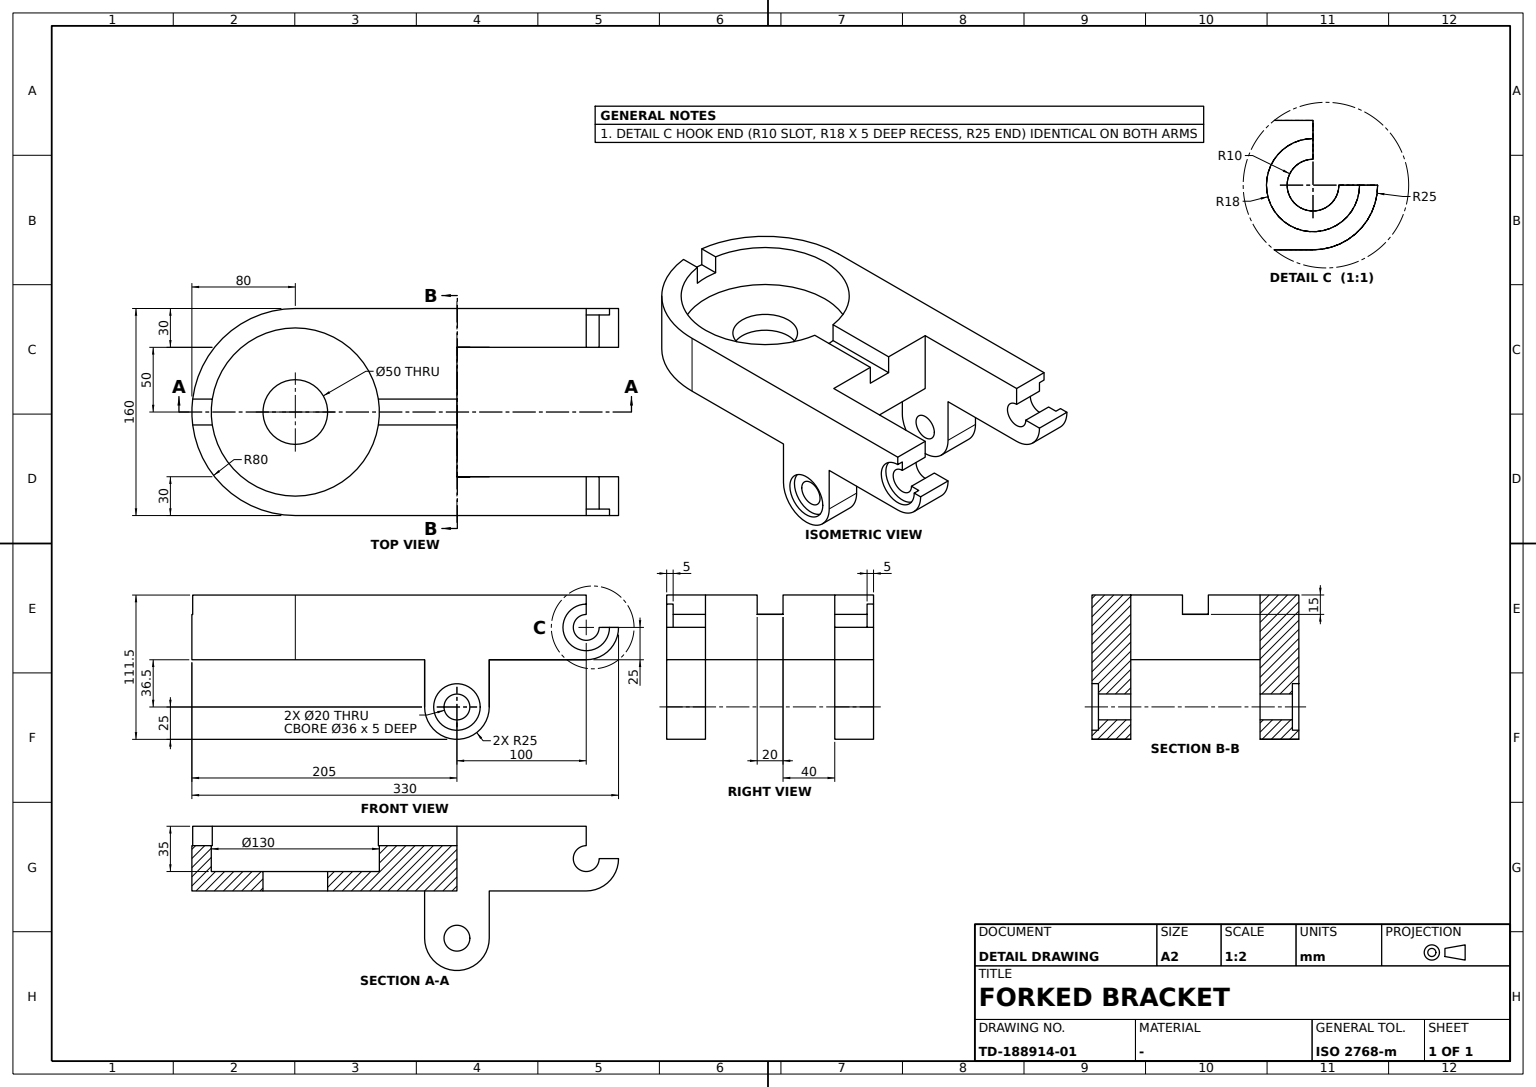
solid
v1 (75,107,25)
v2 (75,143,25)
e1 v1 v2 CIRCLE(AX(P(75,125,25),D(1,0,0),D(0,1,0)),18)
v3 (80,107,25)
e2 v3 v1 LINE
v4 (80,143,25)
e3 v3 v4 CIRCLE(AX(P(80,125,25),D(1,0,0),D(0,1,0)),18)
e4 v4 v2 LINE
face CYL(AX(P(77.5,125,25),D(-1,0,0),D(0,1,0)),18) rev [-e1 -e2 e3 e4]
v5 (-80,0,-36.5)
v6 (-80,50,-36.5)
e5 v5 v6 CIRCLE(AX(P(-80,25,-36.5),D(1,0,0),D(0,1,0)),25)
v7 (-50,50,-36.5)
e6 v6 v7 LINE
v8 (-50,0,-36.5)
e7 v7 v8 CIRCLE(AX(P(-50,25,-36.5),D(-1,0,0),D(0,1,0)),25)
e8 v5 v8 LINE
face CYL(AX(P(0,25,-36.5),D(-1,0,0),D(0,1,0)),25) [e5 e6 e7 -e8]
v9 (-80,125,43)
v10 (-80,125,50)
e9 v9 v10 LINE
v11 (-50,125,50)
e10 v11 v10 LINE
v12 (-50,125,35)
e11 v12 v11 LINE
v13 (-75,125,35)
e12 v12 v13 LINE
v14 (-75,125,43)
e13 v13 v14 LINE
e14 v14 v9 LINE
face PLANE(AX(P(80,125,25),D(0,-1,0),D(0,0,1))) rev [e9 -e10 -e11 e12 e13 e14]
v15 (-25,-100.000066,15)
v16 (-25,-100.000066,0)
e15 v15 v16 LINE
v17 (25,-100.000066,15)
e16 v15 v17 CIRCLE(AX(P(0,-100.000066,15),D(0,0,1),D(1,0,0)),25)
v18 (25,-100.000066,0)
e17 v17 v18 LINE
e18 v18 v16 CIRCLE(AX(P(0,-100.000066,0),D(0,0,-1),D(0,1,0)),25)
face CYL(AX(P(0,-100.000066,-2.5),D(0,0,-1),D(1,0,0)),25) rev [-e15 e16 e17 e18]
v19 (-50,50,0)
v20 (-50,125,0)
e19 v19 v20 LINE
v21 (-80,50,0)
e20 v21 v19 LINE
v22 (-80,125,0)
e21 v21 v22 LINE
e22 v20 v22 LINE
face PLANE(AX(P(0,50,0),D(0,0,-1),D(0,1,0))) [-e19 -e20 e21 -e22]
v23 (-80,107,25)
v24 (-80,143,25)
e23 v23 v24 CIRCLE(AX(P(-80,125,25),D(1,0,0),D(0,1,0)),18)
v25 (-75,107,25)
e24 v23 v25 LINE
v26 (-75,143,25)
e25 v25 v26 CIRCLE(AX(P(-75,125,25),D(1,0,0),D(0,1,0)),18)
e26 v24 v26 LINE
face CYL(AX(P(77.5,125,25),D(-1,0,0),D(0,1,0)),18) rev [-e23 e24 e25 -e26]
v27 (-80,150,25)
e27 v24 v27 LINE
v28 (-75,135,25)
e28 v28 v26 LINE
v29 (-50,135,25)
e29 v29 v28 LINE
v30 (-50,150,25)
e30 v29 v30 LINE
e31 v27 v30 LINE
face PLANE(AX(P(80,125,25),D(0,0,1),D(0,1,0))) [-e27 e26 -e28 -e29 e30 -e31]
v31 (75,15,-36.5)
v32 (50,15,-36.5)
e32 v31 v32 LINE
v33 (50,35,-36.5)
e33 v33 v32 CIRCLE(AX(P(50,25,-36.5),D(1,0,0),D(0,-1,0)),10)
v34 (75,35,-36.5)
e34 v34 v33 LINE
e35 v34 v31 CIRCLE(AX(P(75,25,-36.5),D(1,0,0),D(0,1,0)),10)
face CYL(AX(P(-0.66,25,-36.5),D(-1,0,0),D(0,1,0)),10) rev [e32 -e33 -e34 e35]
e36 v14 v25 CIRCLE(AX(P(-75,125,25),D(1,0,0),D(0,1,0)),18)
e37 v9 v23 CIRCLE(AX(P(-80,125,25),D(1,0,0),D(0,1,0)),18)
face CYL(AX(P(77.5,125,25),D(-1,0,0),D(0,1,0)),18) rev [e36 -e24 -e37 -e14]
v35 (-75,115,25)
e38 v35 v28 CIRCLE(AX(P(-75,125,25),D(1,0,0),D(0,1,0)),10)
v36 (-50,115,25)
e39 v36 v35 LINE
e40 v29 v36 CIRCLE(AX(P(-50,125,25),D(-1,0,0),D(0,1,0)),10)
face CYL(AX(P(-3.16,125,25),D(-1,0,0),D(0,1,0)),10) rev [-e38 -e39 -e40 e29]
v37 (75,115,25)
v38 (50,115,25)
e41 v37 v38 LINE
v39 (75,135,25)
e42 v37 v39 CIRCLE(AX(P(75,125,25),D(1,0,0),D(0,1,0)),10)
v40 (50,135,25)
e43 v39 v40 LINE
e44 v38 v40 CIRCLE(AX(P(50,125,25),D(1,0,0),D(0,-1,0)),10)
face CYL(AX(P(-3.16,125,25),D(-1,0,0),D(0,1,0)),10) rev [-e41 e42 e43 -e44]
e45 v13 v35 CIRCLE(AX(P(-75,125,25),D(1,0,0),D(0,1,0)),10)
face PLANE(AX(P(-75,0,0),D(1,0,0),D(0,1,0))) rev [-e36 -e13 e45 e38 e28 -e25]
e46 v16 v18 CIRCLE(AX(P(0,-100.000066,0),D(0,0,-1),D(0,1,0)),25)
v41 (50,25,0)
v42 (50,0,0)
e47 v41 v42 LINE
v43 (80,0,0)
e48 v42 v43 LINE
v44 (80,-100,0)
e49 v44 v43 LINE
v45 (80,-100.000066,0)
e50 v45 v44 CIRCLE(AX(P(0,-100.000066,0),D(0,0,1),D(1,0,0)),80)
v46 (-80,-100.000066,0)
e51 v46 v45 CIRCLE(AX(P(0,-100.000066,0),D(0,0,1),D(1,0,0)),80)
v47 (-80,-100,0)
e52 v47 v46 CIRCLE(AX(P(0,-100.000066,0),D(0,0,1),D(1,0,0)),80)
v48 (-80,0,0)
e53 v47 v48 LINE
v49 (-50,0,0)
e54 v48 v49 LINE
v50 (-50,25,0)
e55 v50 v49 LINE
e56 v50 v41 LINE
face PLANE(AX(P(0,50,0),D(0,0,-1),D(0,1,0))) [-e18 -e46] [e47 e48 -e49 -e50 -e51 -e52 e53 e54 -e55 e56]
e57 v7 v19 LINE
e58 v6 v21 LINE
face PLANE(AX(P(0,50,-36.5),D(0,1,0),D(0,0,1))) [-e57 -e6 e58 e20]
e59 v32 v33 CIRCLE(AX(P(50,25,-36.5),D(1,0,0),D(0,-1,0)),10)
v51 (50,125,0)
v52 (50,150,25)
e60 v51 v52 CIRCLE(AX(P(50,125,25),D(1,0,0),D(0,1,0)),25)
v53 (50,50,0)
e61 v53 v51 LINE
v54 (50,50,-36.5)
e62 v54 v53 LINE
v55 (50,0,-36.5)
e63 v55 v54 CIRCLE(AX(P(50,25,-36.5),D(1,0,0),D(0,-1,0)),25)
e64 v42 v55 LINE
v56 (50,25,50)
e65 v56 v41 LINE
v57 (50,125,50)
e66 v56 v57 LINE
v58 (50,125,35)
e67 v58 v57 LINE
e68 v58 v38 CIRCLE(AX(P(50,125,25),D(1,0,0),D(0,-1,0)),10)
e69 v40 v52 LINE
face PLANE(AX(P(50,128.473083,50),D(1,0,0),D(0,-1,0))) rev [e59 e33] [-e60 -e61 -e62 -e63 -e64 -e47 -e65 e66 -e67 e68 e44 e69]
v59 (-75,43,-36.5)
v60 (-75,7,-36.5)
e70 v59 v60 CIRCLE(AX(P(-75,25,-36.5),D(1,0,0),D(0,1,0)),18)
v61 (-80,7,-36.5)
e71 v61 v60 LINE
v62 (-80,43,-36.5)
e72 v62 v61 CIRCLE(AX(P(-80,25,-36.5),D(1,0,0),D(0,1,0)),18)
e73 v62 v59 LINE
face CYL(AX(P(77.5,25,-36.5),D(-1,0,0),D(0,1,0)),18) rev [e70 -e71 -e72 e73]
v63 (80,50,-36.5)
e74 v54 v63 LINE
v64 (80,0,-36.5)
e75 v64 v63 CIRCLE(AX(P(80,25,-36.5),D(1,0,0),D(0,1,0)),25)
e76 v55 v64 LINE
face CYL(AX(P(0,25,-36.5),D(-1,0,0),D(0,1,0)),25) [e63 e74 -e75 -e76]
v65 (-50,15,-36.5)
v66 (-50,35,-36.5)
e77 v65 v66 CIRCLE(AX(P(-50,25,-36.5),D(-1,0,0),D(0,1,0)),10)
e78 v66 v65 CIRCLE(AX(P(-50,25,-36.5),D(-1,0,0),D(0,1,0)),10)
e79 v49 v8 LINE
e80 v20 v30 CIRCLE(AX(P(-50,125,25),D(1,0,0),D(0,1,0)),25)
e81 v36 v12 CIRCLE(AX(P(-50,125,25),D(-1,0,0),D(0,1,0)),10)
v67 (-50,25,50)
e82 v11 v67 LINE
e83 v67 v50 LINE
face PLANE(AX(P(-50,25,50),D(-1,0,0),D(0,1,0))) rev [e77 e78] [e55 e79 -e7 e57 e19 e80 -e30 e40 e81 e11 e82 e83]
v68 (-75,15,-36.5)
v69 (-75,35,-36.5)
e84 v68 v69 CIRCLE(AX(P(-75,25,-36.5),D(1,0,0),D(0,1,0)),10)
e85 v65 v68 LINE
e86 v66 v69 LINE
face CYL(AX(P(-0.66,25,-36.5),D(-1,0,0),D(0,1,0)),10) rev [-e84 -e85 -e78 e86]
e87 v22 v27 CIRCLE(AX(P(-80,125,25),D(1,0,0),D(0,1,0)),25)
e88 v48 v5 LINE
v70 (-80,-100,50)
e89 v70 v47 LINE
e90 v10 v70 LINE
e91 v61 v62 CIRCLE(AX(P(-80,25,-36.5),D(1,0,0),D(0,1,0)),18)
face PLANE(AX(P(-80,0,0),D(1,0,0),D(0,1,0))) rev [-e87 -e21 -e58 -e5 -e88 -e53 -e89 -e90 -e9 e37 e23 e27] [e72 e91]
v71 (-80,-100.000066,50)
e92 v70 v71 CIRCLE(AX(P(0,-100.000066,50),D(0,0,1),D(1,0,0)),80)
v72 (-10,-179.372605,50)
e93 v71 v72 CIRCLE(AX(P(0,-100.000066,50),D(0,0,1),D(1,0,0)),80)
v73 (-10,-164.226229,50)
e94 v73 v72 LINE
v74 (-65,-100.000066,50)
e95 v74 v73 CIRCLE(AX(P(0,-100.000066,50),D(0,0,1),D(1,0,0)),65)
v75 (-10,-35.773903,50)
e96 v75 v74 CIRCLE(AX(P(0,-100.000066,50),D(0,0,1),D(1,0,0)),65)
v76 (-10,25,50)
e97 v76 v75 LINE
e98 v67 v76 LINE
face PLANE(AX(P(0,-100,50),D(0,0,-1),D(0,1,0))) rev [e90 e92 e93 -e94 -e95 -e96 -e97 -e98 -e82 e10]
face CYL(AX(P(-3.16,125,25),D(-1,0,0),D(0,1,0)),10) rev [e39 -e45 -e12 -e81]
v77 (10,-179.372605,50)
v78 (10,-164.226229,50)
e99 v77 v78 LINE
v79 (80,-100.000066,50)
e100 v77 v79 CIRCLE(AX(P(0,-100.000066,50),D(0,0,1),D(1,0,0)),80)
v80 (80,-100,50)
e101 v79 v80 CIRCLE(AX(P(0,-100.000066,50),D(0,0,1),D(1,0,0)),80)
v81 (80,125,50)
e102 v81 v80 LINE
e103 v57 v81 LINE
v82 (10,25,50)
e104 v82 v56 LINE
v83 (10,-35.773903,50)
e105 v83 v82 LINE
v84 (65,-100.000066,50)
e106 v84 v83 CIRCLE(AX(P(0,-100.000066,50),D(0,0,1),D(1,0,0)),65)
e107 v78 v84 CIRCLE(AX(P(0,-100.000066,50),D(0,0,1),D(1,0,0)),65)
face PLANE(AX(P(0,-100,50),D(0,0,-1),D(0,1,0))) rev [-e99 e100 e101 -e102 -e103 -e66 -e104 -e105 -e106 -e107]
e108 v69 v68 CIRCLE(AX(P(-75,25,-36.5),D(1,0,0),D(0,1,0)),10)
e109 v60 v59 CIRCLE(AX(P(-75,25,-36.5),D(1,0,0),D(0,1,0)),18)
face PLANE(AX(P(-75,0,0),D(1,0,0),D(0,1,0))) rev [e84 e108] [-e70 -e109]
e110 v71 v46 LINE
face CYL(AX(P(0,-100.000066,25),D(0,0,-1),D(1,0,0)),80) [-e92 e89 e52 -e110]
e111 v79 v45 LINE
v85 (10,-179.372605,35)
e112 v77 v85 LINE
v86 (-10,-179.372605,35)
e113 v86 v85 CIRCLE(AX(P(0,-100.000066,35),D(0,0,1),D(1,0,0)),80)
e114 v72 v86 LINE
face CYL(AX(P(0,-100.000066,25),D(0,0,-1),D(1,0,0)),80) [e51 -e111 -e100 e112 -e113 -e114 -e93 e110]
e115 v17 v15 CIRCLE(AX(P(0,-100.000066,15),D(0,0,1),D(1,0,0)),25)
face CYL(AX(P(0,-100.000066,-2.5),D(0,0,-1),D(1,0,0)),25) rev [e115 e15 e46 -e17]
v87 (10,-164.226229,35)
e116 v85 v87 LINE
v88 (-10,-164.226229,35)
e117 v88 v87 CIRCLE(AX(P(0,-100.000066,35),D(0,0,1),D(1,0,0)),65)
e118 v88 v86 LINE
face PLANE(AX(P(0,0,35),D(0,0,1),D(1,0,0))) [e113 e116 -e117 e118]
e119 v78 v87 LINE
face PLANE(AX(P(10,25,50),D(1,0,0),D(0,-1,0))) rev [-e112 e99 e119 -e116]
v89 (80,125,0)
e120 v51 v89 LINE
v90 (80,50,0)
e121 v90 v89 LINE
e122 v53 v90 LINE
face PLANE(AX(P(0,50,0),D(0,0,-1),D(0,1,0))) [e61 e120 -e121 -e122]
face PLANE(AX(P(0,0,0),D(0,-1,0),D(0,0,-1))) [-e79 -e54 e88 e8]
v91 (80,150,25)
e123 v91 v52 LINE
e124 v39 v2 LINE
e125 v4 v91 LINE
face PLANE(AX(P(80,125,25),D(0,0,1),D(0,1,0))) [e123 -e69 -e43 e124 -e4 e125]
v92 (10,25,35)
e126 v82 v92 LINE
v93 (10,-35.773903,35)
e127 v93 v92 LINE
e128 v83 v93 LINE
face PLANE(AX(P(10,25,50),D(1,0,0),D(0,-1,0))) rev [e105 e126 -e127 -e128]
v94 (80,125,43)
v95 (75,125,43)
e129 v94 v95 LINE
e130 v94 v3 CIRCLE(AX(P(80,125,25),D(1,0,0),D(0,1,0)),18)
e131 v95 v1 CIRCLE(AX(P(75,125,25),D(1,0,0),D(0,1,0)),18)
face CYL(AX(P(77.5,125,25),D(-1,0,0),D(0,1,0)),18) rev [-e129 e130 e2 -e131]
v96 (75,125,35)
e132 v96 v37 CIRCLE(AX(P(75,125,25),D(1,0,0),D(0,1,0)),10)
e133 v96 v95 LINE
face PLANE(AX(P(75,0,0),D(1,0,0),D(0,1,0))) [e131 e1 -e124 -e42 -e132 e133]
e134 v63 v90 LINE
e135 v89 v91 CIRCLE(AX(P(80,125,25),D(1,0,0),D(0,1,0)),25)
e136 v81 v94 LINE
e137 v80 v44 LINE
e138 v43 v64 LINE
v97 (80,7,-36.5)
v98 (80,43,-36.5)
e139 v97 v98 CIRCLE(AX(P(80,25,-36.5),D(1,0,0),D(0,1,0)),18)
e140 v98 v97 CIRCLE(AX(P(80,25,-36.5),D(1,0,0),D(0,1,0)),18)
face PLANE(AX(P(80,0,0),D(1,0,0),D(0,1,0))) [e75 e134 e121 e135 -e125 -e3 -e130 -e136 e102 e137 e49 e138] [-e139 -e140]
e141 v73 v88 LINE
face PLANE(AX(P(-10,-203.24811,50),D(-1,0,0),D(0,1,0))) rev [e114 -e118 -e141 e94]
v99 (-65,-100.000066,15)
e142 v74 v99 LINE
v100 (65,-100.000066,15)
e143 v100 v99 CIRCLE(AX(P(0,-100.000066,15),D(0,0,1),D(1,0,0)),65)
e144 v84 v100 LINE
v101 (-10,-35.773903,35)
e145 v93 v101 CIRCLE(AX(P(0,-100.000066,35),D(0,0,1),D(1,0,0)),65)
e146 v75 v101 LINE
face CYL(AX(P(0,-100.000066,32.5),D(0,0,-1),D(1,0,0)),65) rev [e142 -e143 -e144 e106 e128 e145 -e146 e96]
face CYL(AX(P(77.5,25,-36.5),D(-1,0,0),D(0,1,0)),18) rev [e71 e109 -e73 -e91]
face PLANE(AX(P(0,50,-36.5),D(0,1,0),D(0,0,1))) [e62 e122 -e134 -e74]
e147 v99 v100 CIRCLE(AX(P(0,-100.000066,15),D(0,0,1),D(1,0,0)),65)
face CYL(AX(P(0,-100.000066,32.5),D(0,0,-1),D(1,0,0)),65) rev [-e142 e95 e141 e117 -e119 e107 e144 -e147]
face CYL(AX(P(0,-100.000066,25),D(0,0,-1),D(1,0,0)),80) [e50 -e137 -e101 e111]
v102 (-10,25,35)
e148 v92 v102 LINE
e149 v102 v101 LINE
face PLANE(AX(P(0,0,35),D(0,0,1),D(1,0,0))) [e148 e149 -e145 e127]
face CYL(AX(P(-0.66,25,-36.5),D(-1,0,0),D(0,1,0)),10) rev [e85 -e108 -e86 -e77]
face CYL(AX(P(65,125,25),D(-1,0,0),D(0,1,0)),25) [-e120 e60 -e123 -e135]
e150 v96 v58 LINE
face CYL(AX(P(-3.16,125,25),D(-1,0,0),D(0,1,0)),10) rev [e41 -e68 -e150 e132]
v103 (75,7,-36.5)
v104 (75,43,-36.5)
e151 v103 v104 CIRCLE(AX(P(75,25,-36.5),D(1,0,0),D(0,1,0)),18)
e152 v104 v103 CIRCLE(AX(P(75,25,-36.5),D(1,0,0),D(0,1,0)),18)
e153 v31 v34 CIRCLE(AX(P(75,25,-36.5),D(1,0,0),D(0,1,0)),10)
face PLANE(AX(P(75,0,0),D(1,0,0),D(0,1,0))) [e151 e152] [-e35 -e153]
e154 v76 v102 LINE
face PLANE(AX(P(-10,-203.24811,50),D(-1,0,0),D(0,1,0))) rev [-e154 e97 e146 -e149]
face PLANE(AX(P(-10,25,50),D(0,1,0),D(1,0,0))) [e65 -e56 -e83 e98 e154 -e148 -e126 e104]
face PLANE(AX(P(80,125,25),D(0,-1,0),D(0,0,1))) rev [e129 -e133 e150 e67 e103 e136]
face PLANE(AX(P(0,0,15),D(0,0,1),D(1,0,0))) [-e16 -e115] [e147 e143]
e155 v98 v104 LINE
e156 v97 v103 LINE
face CYL(AX(P(77.5,25,-36.5),D(-1,0,0),D(0,1,0)),18) rev [e139 e155 -e151 -e156]
face CYL(AX(P(-0.66,25,-36.5),D(-1,0,0),D(0,1,0)),10) rev [e153 e34 -e59 -e32]
face CYL(AX(P(65,125,25),D(-1,0,0),D(0,1,0)),25) [e31 -e80 e22 e87]
face CYL(AX(P(77.5,25,-36.5),D(-1,0,0),D(0,1,0)),18) rev [e156 -e152 -e155 e140]
face PLANE(AX(P(0,0,0),D(0,-1,0),D(0,0,-1))) [e64 e76 -e138 -e48]
